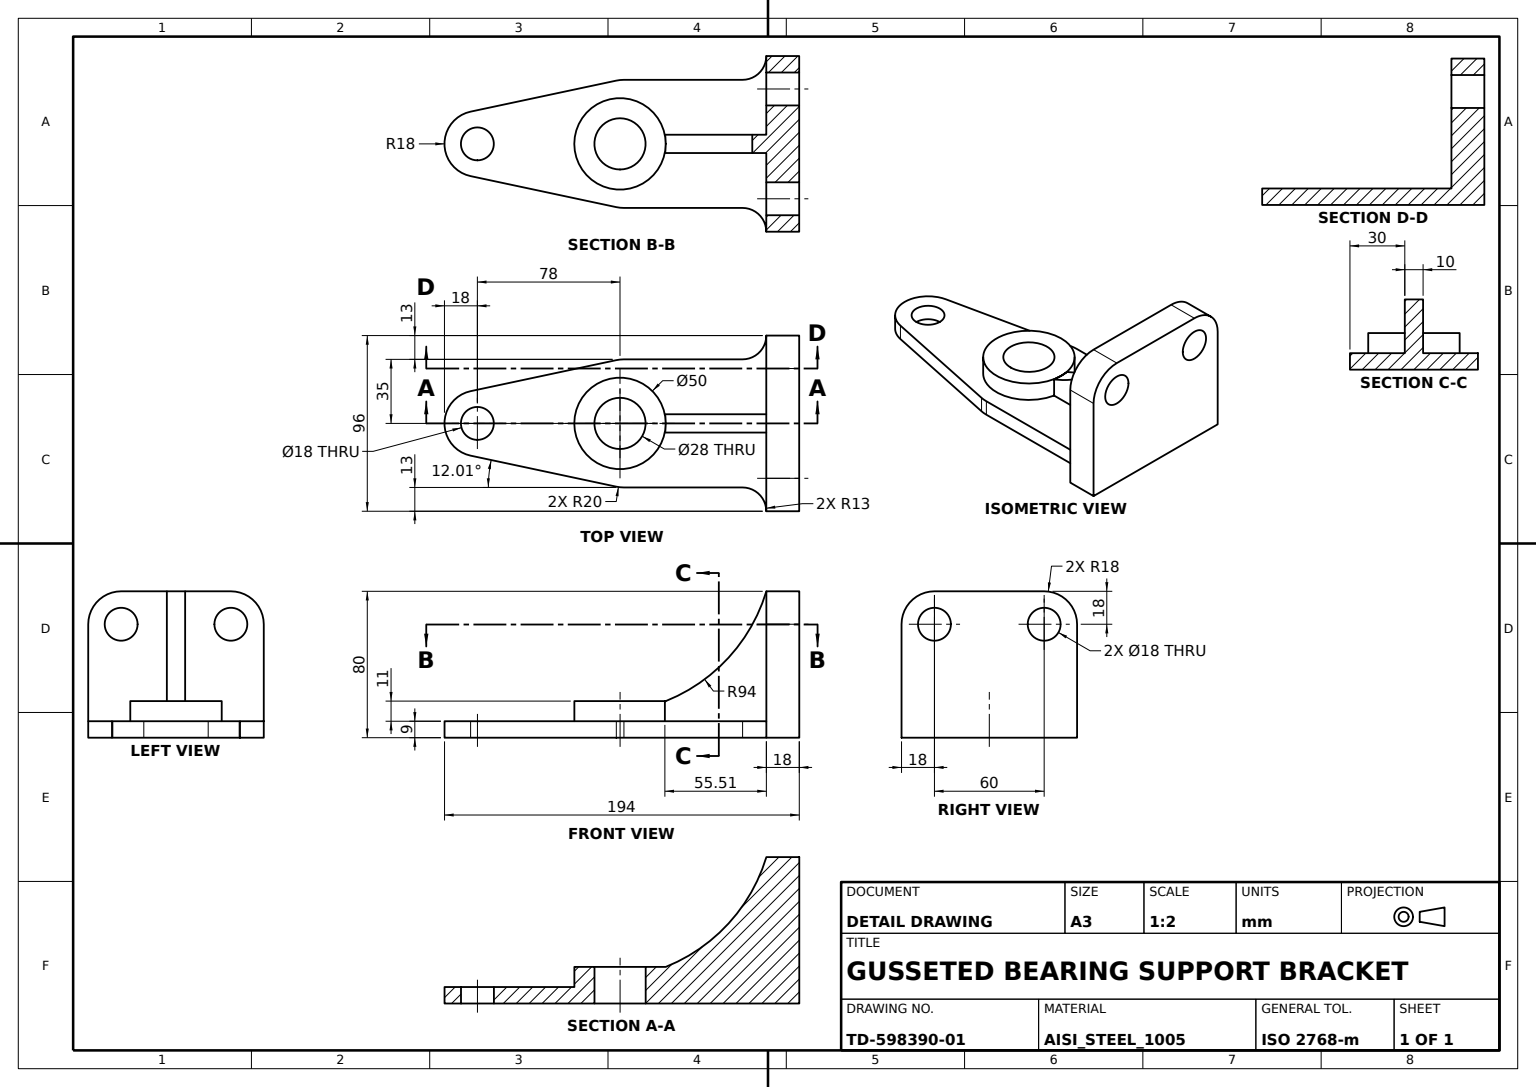
ISO-10303-21;
HEADER;
FILE_DESCRIPTION((''),'2;1');
FILE_NAME('','',(''),(''),'','','');
FILE_SCHEMA(('AUTOMOTIVE_DESIGN'));
ENDSEC;
DATA;
#1=APPLICATION_CONTEXT('');
#2=PRODUCT_CONTEXT('',#1,'mechanical');
#3=PRODUCT('','','',(#2));
#4=PRODUCT_DEFINITION_FORMATION('','',#3);
#5=PRODUCT_DEFINITION_CONTEXT('',#1,'design');
#6=PRODUCT_DEFINITION('','',#4,#5);
#7=PRODUCT_DEFINITION_SHAPE('','',#6);
#8=(LENGTH_UNIT()NAMED_UNIT(*)SI_UNIT(.MILLI.,.METRE.));
#9=(NAMED_UNIT(*)PLANE_ANGLE_UNIT()SI_UNIT($,.RADIAN.));
#10=(NAMED_UNIT(*)SI_UNIT($,.STERADIAN.)SOLID_ANGLE_UNIT());
#11=UNCERTAINTY_MEASURE_WITH_UNIT(LENGTH_MEASURE(0.005),#8,'distance_accuracy_value','');
#12=(GEOMETRIC_REPRESENTATION_CONTEXT(3)GLOBAL_UNCERTAINTY_ASSIGNED_CONTEXT((#11))GLOBAL_UNIT_ASSIGNED_CONTEXT((#8,#9,#10))REPRESENTATION_CONTEXT('',''));
#13=CARTESIAN_POINT('',(9.,0.,9.));
#14=VERTEX_POINT('',#13);
#15=CARTESIAN_POINT('',(0.,0.,9.));
#16=DIRECTION('',(0.,0.,1.));
#17=DIRECTION('',(1.,0.,0.));
#18=AXIS2_PLACEMENT_3D('',#15,#16,#17);
#19=CIRCLE('',#18,9.);
#20=EDGE_CURVE('',#14,#14,#19,.T.);
#21=ORIENTED_EDGE('',*,*,#20,.T.);
#22=EDGE_LOOP('',(#21));
#23=FACE_BOUND('',#22,.T.);
#24=CARTESIAN_POINT('',(9.,0.,0.));
#25=VERTEX_POINT('',#24);
#26=CARTESIAN_POINT('',(0.,0.,0.));
#27=AXIS2_PLACEMENT_3D('',#26,#16,#17);
#28=CIRCLE('',#27,9.);
#29=EDGE_CURVE('',#25,#25,#28,.T.);
#30=ORIENTED_EDGE('',*,*,#29,.F.);
#31=EDGE_LOOP('',(#30));
#32=FACE_BOUND('',#31,.T.);
#33=DIRECTION('',(0.,0.,-1.));
#34=DIRECTION('',(-1.,0.,0.));
#35=AXIS2_PLACEMENT_3D('',#15,#33,#34);
#36=CYLINDRICAL_SURFACE('',#35,9.);
#37=ADVANCED_FACE('',(#23,#32),#36,.F.);
#38=CARTESIAN_POINT('',(-5.,103.,20.));
#39=VERTEX_POINT('',#38);
#40=CARTESIAN_POINT('',(-5.,158.,80.));
#41=VERTEX_POINT('',#40);
#42=CARTESIAN_POINT('',(-5.,68.038419,107.256449));
#43=DIRECTION('',(0.,1.,0.));
#44=AXIS2_PLACEMENT_3D('',#42,#17,#43);
#45=CIRCLE('',#44,94.);
#46=EDGE_CURVE('',#39,#41,#45,.T.);
#47=ORIENTED_EDGE('',*,*,#46,.T.);
#48=CARTESIAN_POINT('',(-5.,158.,9.));
#49=VERTEX_POINT('',#48);
#50=CARTESIAN_POINT('',(-5.,158.,107.256449));
#51=VECTOR('',#16,1000.);
#52=LINE('',#50,#51);
#53=EDGE_CURVE('',#49,#41,#52,.T.);
#54=ORIENTED_EDGE('',*,*,#53,.F.);
#55=CARTESIAN_POINT('',(-5.,102.494897,9.));
#56=VERTEX_POINT('',#55);
#57=CARTESIAN_POINT('',(-5.,68.038419,9.));
#58=VECTOR('',#43,1000.);
#59=LINE('',#57,#58);
#60=EDGE_CURVE('',#56,#49,#59,.T.);
#61=ORIENTED_EDGE('',*,*,#60,.F.);
#62=CARTESIAN_POINT('',(-5.,102.494897,19.797617));
#63=VERTEX_POINT('',#62);
#64=CARTESIAN_POINT('',(-5.,102.494897,20.));
#65=VECTOR('',#33,1000.);
#66=LINE('',#64,#65);
#67=EDGE_CURVE('',#63,#56,#66,.T.);
#68=ORIENTED_EDGE('',*,*,#67,.F.);
#69=DIRECTION('',(0.,-0.928260095,-0.371931709));
#70=VECTOR('',#69,1000.);
#71=LINE('',#38,#70);
#72=EDGE_CURVE('',#39,#63,#71,.T.);
#73=ORIENTED_EDGE('',*,*,#72,.F.);
#74=EDGE_LOOP('',(#47,#54,#61,#68,#73));
#75=FACE_BOUND('',#74,.T.);
#76=AXIS2_PLACEMENT_3D('',#42,#17,#33);
#77=PLANE('',#76);
#78=ADVANCED_FACE('',(#75),#77,.F.);
#79=CARTESIAN_POINT('',(0.,103.,20.));
#80=VERTEX_POINT('',#79);
#81=CARTESIAN_POINT('',(5.,103.,20.));
#82=VECTOR('',#34,1000.);
#83=LINE('',#81,#82);
#84=EDGE_CURVE('',#80,#39,#83,.T.);
#85=ORIENTED_EDGE('',*,*,#84,.F.);
#86=VERTEX_POINT('',#81);
#87=EDGE_CURVE('',#86,#80,#83,.T.);
#88=ORIENTED_EDGE('',*,*,#87,.F.);
#89=CARTESIAN_POINT('',(5.,158.,80.));
#90=VERTEX_POINT('',#89);
#91=CARTESIAN_POINT('',(5.,68.038419,107.256449));
#92=AXIS2_PLACEMENT_3D('',#91,#17,#43);
#93=CIRCLE('',#92,94.);
#94=EDGE_CURVE('',#86,#90,#93,.T.);
#95=ORIENTED_EDGE('',*,*,#94,.T.);
#96=LINE('',#89,#82);
#97=EDGE_CURVE('',#90,#41,#96,.T.);
#98=ORIENTED_EDGE('',*,*,#97,.T.);
#99=ORIENTED_EDGE('',*,*,#46,.F.);
#100=EDGE_LOOP('',(#85,#88,#95,#98,#99));
#101=FACE_BOUND('',#100,.T.);
#102=AXIS2_PLACEMENT_3D('',#91,#34,#16);
#103=CYLINDRICAL_SURFACE('',#102,94.);
#104=ADVANCED_FACE('',(#101),#103,.F.);
#105=CARTESIAN_POINT('',(0.,78.,9.983095));
#106=DIRECTION('',(0.,0.371931709,-0.928260095));
#107=AXIS2_PLACEMENT_3D('',#105,#106,#69);
#108=ELLIPSE('',#107,26.932107,25.);
#109=EDGE_CURVE('',#80,#63,#108,.F.);
#110=ORIENTED_EDGE('',*,*,#109,.F.);
#111=ORIENTED_EDGE('',*,*,#84,.T.);
#112=ORIENTED_EDGE('',*,*,#72,.T.);
#113=EDGE_LOOP('',(#110,#111,#112));
#114=FACE_BOUND('',#113,.T.);
#115=DIRECTION('',(0.,0.928260095,0.371931709));
#116=AXIS2_PLACEMENT_3D('',#81,#106,#115);
#117=PLANE('',#116);
#118=ADVANCED_FACE('',(#114),#117,.F.);
#119=CARTESIAN_POINT('',(-17.605848,-3.746214,9.));
#120=VERTEX_POINT('',#119);
#121=CARTESIAN_POINT('',(-17.605848,-3.746214,0.));
#122=VERTEX_POINT('',#121);
#123=LINE('',#119,#65);
#124=EDGE_CURVE('',#120,#122,#123,.T.);
#125=ORIENTED_EDGE('',*,*,#124,.T.);
#126=CARTESIAN_POINT('',(17.605848,-3.746214,0.));
#127=VERTEX_POINT('',#126);
#128=AXIS2_PLACEMENT_3D('',#26,#33,#17);
#129=CIRCLE('',#128,18.);
#130=EDGE_CURVE('',#127,#122,#129,.T.);
#131=ORIENTED_EDGE('',*,*,#130,.F.);
#132=CARTESIAN_POINT('',(17.605848,-3.746214,9.));
#133=VERTEX_POINT('',#132);
#134=LINE('',#132,#65);
#135=EDGE_CURVE('',#133,#127,#134,.T.);
#136=ORIENTED_EDGE('',*,*,#135,.F.);
#137=AXIS2_PLACEMENT_3D('',#15,#33,#17);
#138=CIRCLE('',#137,18.);
#139=EDGE_CURVE('',#133,#120,#138,.T.);
#140=ORIENTED_EDGE('',*,*,#139,.T.);
#141=EDGE_LOOP('',(#125,#131,#136,#140));
#142=FACE_BOUND('',#141,.T.);
#143=CYLINDRICAL_SURFACE('',#35,18.);
#144=ADVANCED_FACE('',(#142),#143,.T.);
#145=CARTESIAN_POINT('',(48.,176.,0.));
#146=VERTEX_POINT('',#145);
#147=CARTESIAN_POINT('',(48.,158.,0.));
#148=VERTEX_POINT('',#147);
#149=DIRECTION('',(0.,-1.,0.));
#150=VECTOR('',#149,1000.);
#151=LINE('',#145,#150);
#152=EDGE_CURVE('',#146,#148,#151,.T.);
#153=ORIENTED_EDGE('',*,*,#152,.F.);
#154=CARTESIAN_POINT('',(48.,176.,62.));
#155=VERTEX_POINT('',#154);
#156=LINE('',#154,#65);
#157=EDGE_CURVE('',#155,#146,#156,.T.);
#158=ORIENTED_EDGE('',*,*,#157,.F.);
#159=CARTESIAN_POINT('',(48.,158.,62.));
#160=VERTEX_POINT('',#159);
#161=LINE('',#154,#150);
#162=EDGE_CURVE('',#155,#160,#161,.T.);
#163=ORIENTED_EDGE('',*,*,#162,.T.);
#164=CARTESIAN_POINT('',(48.,158.,9.));
#165=VERTEX_POINT('',#164);
#166=LINE('',#159,#65);
#167=EDGE_CURVE('',#160,#165,#166,.T.);
#168=ORIENTED_EDGE('',*,*,#167,.T.);
#169=LINE('',#164,#65);
#170=EDGE_CURVE('',#165,#148,#169,.T.);
#171=ORIENTED_EDGE('',*,*,#170,.T.);
#172=EDGE_LOOP('',(#153,#158,#163,#168,#171));
#173=FACE_BOUND('',#172,.T.);
#174=AXIS2_PLACEMENT_3D('',#154,#34,#16);
#175=PLANE('',#174);
#176=ADVANCED_FACE('',(#173),#175,.F.);
#177=ORIENTED_EDGE('',*,*,#67,.T.);
#178=CARTESIAN_POINT('',(5.,102.494897,9.));
#179=VERTEX_POINT('',#178);
#180=CARTESIAN_POINT('',(0.,78.,9.));
#181=AXIS2_PLACEMENT_3D('',#180,#33,#34);
#182=CIRCLE('',#181,25.);
#183=EDGE_CURVE('',#179,#56,#182,.T.);
#184=ORIENTED_EDGE('',*,*,#183,.F.);
#185=CARTESIAN_POINT('',(5.,102.494897,19.797617));
#186=VERTEX_POINT('',#185);
#187=CARTESIAN_POINT('',(5.,102.494897,20.));
#188=LINE('',#187,#65);
#189=EDGE_CURVE('',#179,#186,#188,.F.);
#190=ORIENTED_EDGE('',*,*,#189,.T.);
#191=EDGE_CURVE('',#186,#80,#108,.F.);
#192=ORIENTED_EDGE('',*,*,#191,.T.);
#193=CARTESIAN_POINT('',(0.,78.,20.));
#194=AXIS2_PLACEMENT_3D('',#193,#33,#17);
#195=CIRCLE('',#194,25.);
#196=EDGE_CURVE('',#80,#80,#195,.T.);
#197=ORIENTED_EDGE('',*,*,#196,.T.);
#198=ORIENTED_EDGE('',*,*,#109,.T.);
#199=EDGE_LOOP('',(#177,#184,#190,#192,#197,#198));
#200=FACE_BOUND('',#199,.T.);
#201=AXIS2_PLACEMENT_3D('',#193,#33,#34);
#202=CYLINDRICAL_SURFACE('',#201,25.);
#203=ADVANCED_FACE('',(#200),#202,.T.);
#204=CARTESIAN_POINT('',(30.,176.,80.));
#205=VERTEX_POINT('',#204);
#206=CARTESIAN_POINT('',(30.,158.,80.));
#207=VERTEX_POINT('',#206);
#208=LINE('',#204,#150);
#209=EDGE_CURVE('',#205,#207,#208,.T.);
#210=ORIENTED_EDGE('',*,*,#209,.T.);
#211=CARTESIAN_POINT('',(30.,158.,62.));
#212=AXIS2_PLACEMENT_3D('',#211,#43,#34);
#213=CIRCLE('',#212,18.);
#214=EDGE_CURVE('',#207,#160,#213,.T.);
#215=ORIENTED_EDGE('',*,*,#214,.T.);
#216=ORIENTED_EDGE('',*,*,#162,.F.);
#217=CARTESIAN_POINT('',(30.,176.,62.));
#218=AXIS2_PLACEMENT_3D('',#217,#43,#34);
#219=CIRCLE('',#218,18.);
#220=EDGE_CURVE('',#205,#155,#219,.T.);
#221=ORIENTED_EDGE('',*,*,#220,.F.);
#222=EDGE_LOOP('',(#210,#215,#216,#221));
#223=FACE_BOUND('',#222,.T.);
#224=AXIS2_PLACEMENT_3D('',#217,#149,#33);
#225=CYLINDRICAL_SURFACE('',#224,18.);
#226=ADVANCED_FACE('',(#223),#225,.T.);
#227=CARTESIAN_POINT('',(14.,78.,0.));
#228=VERTEX_POINT('',#227);
#229=CARTESIAN_POINT('',(0.,78.,0.));
#230=AXIS2_PLACEMENT_3D('',#229,#33,#17);
#231=CIRCLE('',#230,14.);
#232=EDGE_CURVE('',#228,#228,#231,.T.);
#233=ORIENTED_EDGE('',*,*,#232,.F.);
#234=EDGE_LOOP('',(#233));
#235=FACE_BOUND('',#234,.T.);
#236=CARTESIAN_POINT('',(-35.,80.104269,0.));
#237=VERTEX_POINT('',#236);
#238=CARTESIAN_POINT('',(-35.,145.,0.));
#239=VERTEX_POINT('',#238);
#240=LINE('',#236,#58);
#241=EDGE_CURVE('',#237,#239,#240,.T.);
#242=ORIENTED_EDGE('',*,*,#241,.T.);
#243=CARTESIAN_POINT('',(-48.,158.,0.));
#244=VERTEX_POINT('',#243);
#245=CARTESIAN_POINT('',(-48.,145.,0.));
#246=AXIS2_PLACEMENT_3D('',#245,#16,#17);
#247=CIRCLE('',#246,13.);
#248=EDGE_CURVE('',#239,#244,#247,.T.);
#249=ORIENTED_EDGE('',*,*,#248,.T.);
#250=CARTESIAN_POINT('',(-48.,176.,0.));
#251=VERTEX_POINT('',#250);
#252=LINE('',#250,#150);
#253=EDGE_CURVE('',#251,#244,#252,.T.);
#254=ORIENTED_EDGE('',*,*,#253,.F.);
#255=LINE('',#145,#82);
#256=EDGE_CURVE('',#146,#251,#255,.T.);
#257=ORIENTED_EDGE('',*,*,#256,.F.);
#258=ORIENTED_EDGE('',*,*,#152,.T.);
#259=CARTESIAN_POINT('',(35.,145.,0.));
#260=VERTEX_POINT('',#259);
#261=CARTESIAN_POINT('',(48.,145.,0.));
#262=AXIS2_PLACEMENT_3D('',#261,#16,#34);
#263=CIRCLE('',#262,13.);
#264=EDGE_CURVE('',#148,#260,#263,.T.);
#265=ORIENTED_EDGE('',*,*,#264,.T.);
#266=CARTESIAN_POINT('',(35.,80.104269,0.));
#267=VERTEX_POINT('',#266);
#268=LINE('',#259,#150);
#269=EDGE_CURVE('',#260,#267,#268,.T.);
#270=ORIENTED_EDGE('',*,*,#269,.T.);
#271=CARTESIAN_POINT('',(34.562053,75.941809,0.));
#272=VERTEX_POINT('',#271);
#273=CARTESIAN_POINT('',(15.,80.104269,0.));
#274=AXIS2_PLACEMENT_3D('',#273,#33,#34);
#275=CIRCLE('',#274,20.);
#276=EDGE_CURVE('',#267,#272,#275,.T.);
#277=ORIENTED_EDGE('',*,*,#276,.T.);
#278=DIRECTION('',(-0.20812299,-0.978102664,0.));
#279=VECTOR('',#278,1000.);
#280=LINE('',#271,#279);
#281=EDGE_CURVE('',#272,#127,#280,.T.);
#282=ORIENTED_EDGE('',*,*,#281,.T.);
#283=ORIENTED_EDGE('',*,*,#130,.T.);
#284=CARTESIAN_POINT('',(-34.562053,75.941809,0.));
#285=VERTEX_POINT('',#284);
#286=DIRECTION('',(-0.20812299,0.978102664,0.));
#287=VECTOR('',#286,1000.);
#288=LINE('',#121,#287);
#289=EDGE_CURVE('',#122,#285,#288,.T.);
#290=ORIENTED_EDGE('',*,*,#289,.T.);
#291=CARTESIAN_POINT('',(-15.,80.104269,0.));
#292=AXIS2_PLACEMENT_3D('',#291,#33,#17);
#293=CIRCLE('',#292,20.);
#294=EDGE_CURVE('',#285,#237,#293,.T.);
#295=ORIENTED_EDGE('',*,*,#294,.T.);
#296=EDGE_LOOP('',(#242,#249,#254,#257,#258,#265,#270,#277,#282,#283,#290,#295));
#297=FACE_BOUND('',#296,.T.);
#298=ORIENTED_EDGE('',*,*,#29,.T.);
#299=EDGE_LOOP('',(#298));
#300=FACE_BOUND('',#299,.T.);
#301=AXIS2_PLACEMENT_3D('',#26,#33,#34);
#302=PLANE('',#301);
#303=ADVANCED_FACE('',(#235,#297,#300),#302,.T.);
#304=ORIENTED_EDGE('',*,*,#232,.T.);
#305=EDGE_LOOP('',(#304));
#306=FACE_BOUND('',#305,.T.);
#307=CARTESIAN_POINT('',(14.,78.,20.));
#308=VERTEX_POINT('',#307);
#309=CIRCLE('',#194,14.);
#310=EDGE_CURVE('',#308,#308,#309,.T.);
#311=ORIENTED_EDGE('',*,*,#310,.F.);
#312=EDGE_LOOP('',(#311));
#313=FACE_BOUND('',#312,.T.);
#314=CYLINDRICAL_SURFACE('',#201,14.);
#315=ADVANCED_FACE('',(#306,#313),#314,.F.);
#316=CARTESIAN_POINT('',(21.,158.,62.));
#317=VERTEX_POINT('',#316);
#318=CIRCLE('',#212,9.);
#319=EDGE_CURVE('',#317,#317,#318,.T.);
#320=ORIENTED_EDGE('',*,*,#319,.T.);
#321=EDGE_LOOP('',(#320));
#322=FACE_BOUND('',#321,.T.);
#323=ORIENTED_EDGE('',*,*,#167,.F.);
#324=ORIENTED_EDGE('',*,*,#214,.F.);
#325=CARTESIAN_POINT('',(-30.,158.,80.));
#326=VECTOR('',#17,1000.);
#327=LINE('',#325,#326);
#328=EDGE_CURVE('',#90,#207,#327,.T.);
#329=ORIENTED_EDGE('',*,*,#328,.F.);
#330=CARTESIAN_POINT('',(5.,158.,9.));
#331=VERTEX_POINT('',#330);
#332=CARTESIAN_POINT('',(5.,158.,107.256449));
#333=LINE('',#332,#51);
#334=EDGE_CURVE('',#90,#331,#333,.F.);
#335=ORIENTED_EDGE('',*,*,#334,.T.);
#336=CARTESIAN_POINT('',(-48.,158.,9.));
#337=LINE('',#336,#326);
#338=EDGE_CURVE('',#331,#165,#337,.T.);
#339=ORIENTED_EDGE('',*,*,#338,.T.);
#340=EDGE_LOOP('',(#323,#324,#329,#335,#339));
#341=FACE_BOUND('',#340,.T.);
#342=CARTESIAN_POINT('',(-30.,158.,62.));
#343=AXIS2_PLACEMENT_3D('',#342,#43,#16);
#344=PLANE('',#343);
#345=ADVANCED_FACE('',(#322,#341),#344,.F.);
#346=ORIENTED_EDGE('',*,*,#124,.F.);
#347=CARTESIAN_POINT('',(-34.562053,75.941809,9.));
#348=VERTEX_POINT('',#347);
#349=LINE('',#119,#287);
#350=EDGE_CURVE('',#120,#348,#349,.T.);
#351=ORIENTED_EDGE('',*,*,#350,.T.);
#352=LINE('',#347,#65);
#353=EDGE_CURVE('',#348,#285,#352,.T.);
#354=ORIENTED_EDGE('',*,*,#353,.T.);
#355=ORIENTED_EDGE('',*,*,#289,.F.);
#356=EDGE_LOOP('',(#346,#351,#354,#355));
#357=FACE_BOUND('',#356,.T.);
#358=DIRECTION('',(-0.978102664,-0.20812299,0.));
#359=DIRECTION('',(0.20812299,-0.978102664,0.));
#360=AXIS2_PLACEMENT_3D('',#119,#358,#359);
#361=PLANE('',#360);
#362=ADVANCED_FACE('',(#357),#361,.T.);
#363=CARTESIAN_POINT('',(-35.,80.104269,9.));
#364=VERTEX_POINT('',#363);
#365=CARTESIAN_POINT('',(-35.,145.,9.));
#366=VERTEX_POINT('',#365);
#367=LINE('',#363,#58);
#368=EDGE_CURVE('',#364,#366,#367,.T.);
#369=ORIENTED_EDGE('',*,*,#368,.T.);
#370=LINE('',#365,#65);
#371=EDGE_CURVE('',#366,#239,#370,.T.);
#372=ORIENTED_EDGE('',*,*,#371,.T.);
#373=ORIENTED_EDGE('',*,*,#241,.F.);
#374=LINE('',#363,#65);
#375=EDGE_CURVE('',#364,#237,#374,.T.);
#376=ORIENTED_EDGE('',*,*,#375,.F.);
#377=EDGE_LOOP('',(#369,#372,#373,#376));
#378=FACE_BOUND('',#377,.T.);
#379=AXIS2_PLACEMENT_3D('',#363,#34,#149);
#380=PLANE('',#379);
#381=ADVANCED_FACE('',(#378),#380,.T.);
#382=CARTESIAN_POINT('',(35.,145.,9.));
#383=VERTEX_POINT('',#382);
#384=LINE('',#382,#65);
#385=EDGE_CURVE('',#383,#260,#384,.T.);
#386=ORIENTED_EDGE('',*,*,#385,.T.);
#387=ORIENTED_EDGE('',*,*,#264,.F.);
#388=ORIENTED_EDGE('',*,*,#170,.F.);
#389=CARTESIAN_POINT('',(48.,145.,9.));
#390=AXIS2_PLACEMENT_3D('',#389,#16,#34);
#391=CIRCLE('',#390,13.);
#392=EDGE_CURVE('',#165,#383,#391,.T.);
#393=ORIENTED_EDGE('',*,*,#392,.T.);
#394=EDGE_LOOP('',(#386,#387,#388,#393));
#395=FACE_BOUND('',#394,.T.);
#396=AXIS2_PLACEMENT_3D('',#389,#33,#34);
#397=CYLINDRICAL_SURFACE('',#396,13.);
#398=ADVANCED_FACE('',(#395),#397,.F.);
#399=CARTESIAN_POINT('',(-48.,176.,62.));
#400=VERTEX_POINT('',#399);
#401=CARTESIAN_POINT('',(-30.,176.,80.));
#402=VERTEX_POINT('',#401);
#403=CARTESIAN_POINT('',(-30.,176.,62.));
#404=AXIS2_PLACEMENT_3D('',#403,#43,#34);
#405=CIRCLE('',#404,18.);
#406=EDGE_CURVE('',#400,#402,#405,.T.);
#407=ORIENTED_EDGE('',*,*,#406,.F.);
#408=CARTESIAN_POINT('',(-48.,158.,62.));
#409=VERTEX_POINT('',#408);
#410=LINE('',#399,#150);
#411=EDGE_CURVE('',#400,#409,#410,.T.);
#412=ORIENTED_EDGE('',*,*,#411,.T.);
#413=VERTEX_POINT('',#325);
#414=AXIS2_PLACEMENT_3D('',#342,#43,#34);
#415=CIRCLE('',#414,18.);
#416=EDGE_CURVE('',#409,#413,#415,.T.);
#417=ORIENTED_EDGE('',*,*,#416,.T.);
#418=LINE('',#401,#150);
#419=EDGE_CURVE('',#402,#413,#418,.T.);
#420=ORIENTED_EDGE('',*,*,#419,.F.);
#421=EDGE_LOOP('',(#407,#412,#417,#420));
#422=FACE_BOUND('',#421,.T.);
#423=AXIS2_PLACEMENT_3D('',#403,#149,#33);
#424=CYLINDRICAL_SURFACE('',#423,18.);
#425=ADVANCED_FACE('',(#422),#424,.T.);
#426=VERTEX_POINT('',#336);
#427=CARTESIAN_POINT('',(-48.,145.,9.));
#428=AXIS2_PLACEMENT_3D('',#427,#16,#17);
#429=CIRCLE('',#428,13.);
#430=EDGE_CURVE('',#366,#426,#429,.T.);
#431=ORIENTED_EDGE('',*,*,#430,.T.);
#432=LINE('',#336,#65);
#433=EDGE_CURVE('',#426,#244,#432,.T.);
#434=ORIENTED_EDGE('',*,*,#433,.T.);
#435=ORIENTED_EDGE('',*,*,#248,.F.);
#436=ORIENTED_EDGE('',*,*,#371,.F.);
#437=EDGE_LOOP('',(#431,#434,#435,#436));
#438=FACE_BOUND('',#437,.T.);
#439=AXIS2_PLACEMENT_3D('',#427,#33,#34);
#440=CYLINDRICAL_SURFACE('',#439,13.);
#441=ADVANCED_FACE('',(#438),#440,.F.);
#442=ORIENTED_EDGE('',*,*,#385,.F.);
#443=CARTESIAN_POINT('',(35.,80.104269,9.));
#444=VERTEX_POINT('',#443);
#445=LINE('',#382,#150);
#446=EDGE_CURVE('',#383,#444,#445,.T.);
#447=ORIENTED_EDGE('',*,*,#446,.T.);
#448=LINE('',#443,#65);
#449=EDGE_CURVE('',#444,#267,#448,.T.);
#450=ORIENTED_EDGE('',*,*,#449,.T.);
#451=ORIENTED_EDGE('',*,*,#269,.F.);
#452=EDGE_LOOP('',(#442,#447,#450,#451));
#453=FACE_BOUND('',#452,.T.);
#454=AXIS2_PLACEMENT_3D('',#382,#17,#43);
#455=PLANE('',#454);
#456=ADVANCED_FACE('',(#453),#455,.T.);
#457=CARTESIAN_POINT('',(34.562053,75.941809,9.));
#458=VERTEX_POINT('',#457);
#459=LINE('',#457,#279);
#460=EDGE_CURVE('',#458,#133,#459,.T.);
#461=ORIENTED_EDGE('',*,*,#460,.T.);
#462=ORIENTED_EDGE('',*,*,#135,.T.);
#463=ORIENTED_EDGE('',*,*,#281,.F.);
#464=LINE('',#457,#65);
#465=EDGE_CURVE('',#458,#272,#464,.T.);
#466=ORIENTED_EDGE('',*,*,#465,.F.);
#467=EDGE_LOOP('',(#461,#462,#463,#466));
#468=FACE_BOUND('',#467,.T.);
#469=DIRECTION('',(0.978102664,-0.20812299,0.));
#470=DIRECTION('',(0.20812299,0.978102664,0.));
#471=AXIS2_PLACEMENT_3D('',#457,#469,#470);
#472=PLANE('',#471);
#473=ADVANCED_FACE('',(#468),#472,.T.);
#474=ORIENTED_EDGE('',*,*,#310,.T.);
#475=EDGE_LOOP('',(#474));
#476=FACE_BOUND('',#475,.T.);
#477=ORIENTED_EDGE('',*,*,#196,.F.);
#478=EDGE_LOOP('',(#477));
#479=FACE_BOUND('',#478,.T.);
#480=PLANE('',#201);
#481=ADVANCED_FACE('',(#476,#479),#480,.F.);
#482=CARTESIAN_POINT('',(21.,176.,62.));
#483=VERTEX_POINT('',#482);
#484=CIRCLE('',#218,9.);
#485=EDGE_CURVE('',#483,#483,#484,.T.);
#486=ORIENTED_EDGE('',*,*,#485,.F.);
#487=EDGE_LOOP('',(#486));
#488=FACE_BOUND('',#487,.T.);
#489=ORIENTED_EDGE('',*,*,#220,.T.);
#490=ORIENTED_EDGE('',*,*,#157,.T.);
#491=ORIENTED_EDGE('',*,*,#256,.T.);
#492=LINE('',#250,#51);
#493=EDGE_CURVE('',#251,#400,#492,.T.);
#494=ORIENTED_EDGE('',*,*,#493,.T.);
#495=ORIENTED_EDGE('',*,*,#406,.T.);
#496=LINE('',#401,#326);
#497=EDGE_CURVE('',#402,#205,#496,.T.);
#498=ORIENTED_EDGE('',*,*,#497,.T.);
#499=EDGE_LOOP('',(#489,#490,#491,#494,#495,#498));
#500=FACE_BOUND('',#499,.T.);
#501=CARTESIAN_POINT('',(-21.,176.,62.));
#502=VERTEX_POINT('',#501);
#503=AXIS2_PLACEMENT_3D('',#403,#149,#17);
#504=CIRCLE('',#503,9.);
#505=EDGE_CURVE('',#502,#502,#504,.T.);
#506=ORIENTED_EDGE('',*,*,#505,.T.);
#507=EDGE_LOOP('',(#506));
#508=FACE_BOUND('',#507,.T.);
#509=AXIS2_PLACEMENT_3D('',#403,#43,#16);
#510=PLANE('',#509);
#511=ADVANCED_FACE('',(#488,#500,#508),#510,.T.);
#512=LINE('',#81,#70);
#513=EDGE_CURVE('',#86,#186,#512,.T.);
#514=ORIENTED_EDGE('',*,*,#513,.F.);
#515=ORIENTED_EDGE('',*,*,#87,.T.);
#516=ORIENTED_EDGE('',*,*,#191,.F.);
#517=EDGE_LOOP('',(#514,#515,#516));
#518=FACE_BOUND('',#517,.T.);
#519=ADVANCED_FACE('',(#518),#117,.F.);
#520=ORIENTED_EDGE('',*,*,#319,.F.);
#521=EDGE_LOOP('',(#520));
#522=FACE_BOUND('',#521,.T.);
#523=ORIENTED_EDGE('',*,*,#485,.T.);
#524=EDGE_LOOP('',(#523));
#525=FACE_BOUND('',#524,.T.);
#526=CYLINDRICAL_SURFACE('',#224,9.);
#527=ADVANCED_FACE('',(#522,#525),#526,.F.);
#528=ORIENTED_EDGE('',*,*,#449,.F.);
#529=CARTESIAN_POINT('',(15.,80.104269,9.));
#530=AXIS2_PLACEMENT_3D('',#529,#33,#34);
#531=CIRCLE('',#530,20.);
#532=EDGE_CURVE('',#444,#458,#531,.T.);
#533=ORIENTED_EDGE('',*,*,#532,.T.);
#534=ORIENTED_EDGE('',*,*,#465,.T.);
#535=ORIENTED_EDGE('',*,*,#276,.F.);
#536=EDGE_LOOP('',(#528,#533,#534,#535));
#537=FACE_BOUND('',#536,.T.);
#538=CYLINDRICAL_SURFACE('',#530,20.);
#539=ADVANCED_FACE('',(#537),#538,.T.);
#540=LINE('',#243,#51);
#541=EDGE_CURVE('',#426,#409,#540,.T.);
#542=ORIENTED_EDGE('',*,*,#541,.T.);
#543=ORIENTED_EDGE('',*,*,#411,.F.);
#544=ORIENTED_EDGE('',*,*,#493,.F.);
#545=ORIENTED_EDGE('',*,*,#253,.T.);
#546=ORIENTED_EDGE('',*,*,#433,.F.);
#547=EDGE_LOOP('',(#542,#543,#544,#545,#546));
#548=FACE_BOUND('',#547,.T.);
#549=AXIS2_PLACEMENT_3D('',#250,#17,#33);
#550=PLANE('',#549);
#551=ADVANCED_FACE('',(#548),#550,.F.);
#552=ORIENTED_EDGE('',*,*,#419,.T.);
#553=EDGE_CURVE('',#413,#41,#327,.T.);
#554=ORIENTED_EDGE('',*,*,#553,.T.);
#555=ORIENTED_EDGE('',*,*,#97,.F.);
#556=ORIENTED_EDGE('',*,*,#328,.T.);
#557=ORIENTED_EDGE('',*,*,#209,.F.);
#558=ORIENTED_EDGE('',*,*,#497,.F.);
#559=EDGE_LOOP('',(#552,#554,#555,#556,#557,#558));
#560=FACE_BOUND('',#559,.T.);
#561=AXIS2_PLACEMENT_3D('',#401,#33,#34);
#562=PLANE('',#561);
#563=ADVANCED_FACE('',(#560),#562,.F.);
#564=ORIENTED_EDGE('',*,*,#20,.F.);
#565=EDGE_LOOP('',(#564));
#566=FACE_BOUND('',#565,.T.);
#567=ORIENTED_EDGE('',*,*,#139,.F.);
#568=ORIENTED_EDGE('',*,*,#460,.F.);
#569=ORIENTED_EDGE('',*,*,#532,.F.);
#570=ORIENTED_EDGE('',*,*,#446,.F.);
#571=ORIENTED_EDGE('',*,*,#392,.F.);
#572=ORIENTED_EDGE('',*,*,#338,.F.);
#573=CARTESIAN_POINT('',(5.,68.038419,9.));
#574=LINE('',#573,#58);
#575=EDGE_CURVE('',#331,#179,#574,.F.);
#576=ORIENTED_EDGE('',*,*,#575,.T.);
#577=ORIENTED_EDGE('',*,*,#183,.T.);
#578=ORIENTED_EDGE('',*,*,#60,.T.);
#579=EDGE_CURVE('',#426,#49,#337,.T.);
#580=ORIENTED_EDGE('',*,*,#579,.F.);
#581=ORIENTED_EDGE('',*,*,#430,.F.);
#582=ORIENTED_EDGE('',*,*,#368,.F.);
#583=CARTESIAN_POINT('',(-15.,80.104269,9.));
#584=AXIS2_PLACEMENT_3D('',#583,#33,#17);
#585=CIRCLE('',#584,20.);
#586=EDGE_CURVE('',#348,#364,#585,.T.);
#587=ORIENTED_EDGE('',*,*,#586,.F.);
#588=ORIENTED_EDGE('',*,*,#350,.F.);
#589=EDGE_LOOP('',(#567,#568,#569,#570,#571,#572,#576,#577,#578,#580,#581,#582,#587,#588));
#590=FACE_BOUND('',#589,.T.);
#591=PLANE('',#35);
#592=ADVANCED_FACE('',(#566,#590),#591,.F.);
#593=ORIENTED_EDGE('',*,*,#94,.F.);
#594=ORIENTED_EDGE('',*,*,#513,.T.);
#595=ORIENTED_EDGE('',*,*,#189,.F.);
#596=ORIENTED_EDGE('',*,*,#575,.F.);
#597=ORIENTED_EDGE('',*,*,#334,.F.);
#598=EDGE_LOOP('',(#593,#594,#595,#596,#597));
#599=FACE_BOUND('',#598,.T.);
#600=AXIS2_PLACEMENT_3D('',#91,#17,#33);
#601=PLANE('',#600);
#602=ADVANCED_FACE('',(#599),#601,.T.);
#603=ORIENTED_EDGE('',*,*,#505,.F.);
#604=EDGE_LOOP('',(#603));
#605=FACE_BOUND('',#604,.T.);
#606=CARTESIAN_POINT('',(-21.,158.,62.));
#607=VERTEX_POINT('',#606);
#608=AXIS2_PLACEMENT_3D('',#342,#149,#17);
#609=CIRCLE('',#608,9.);
#610=EDGE_CURVE('',#607,#607,#609,.T.);
#611=ORIENTED_EDGE('',*,*,#610,.T.);
#612=EDGE_LOOP('',(#611));
#613=FACE_BOUND('',#612,.T.);
#614=CYLINDRICAL_SURFACE('',#423,9.);
#615=ADVANCED_FACE('',(#605,#613),#614,.F.);
#616=ORIENTED_EDGE('',*,*,#610,.F.);
#617=EDGE_LOOP('',(#616));
#618=FACE_BOUND('',#617,.T.);
#619=ORIENTED_EDGE('',*,*,#53,.T.);
#620=ORIENTED_EDGE('',*,*,#553,.F.);
#621=ORIENTED_EDGE('',*,*,#416,.F.);
#622=ORIENTED_EDGE('',*,*,#541,.F.);
#623=ORIENTED_EDGE('',*,*,#579,.T.);
#624=EDGE_LOOP('',(#619,#620,#621,#622,#623));
#625=FACE_BOUND('',#624,.T.);
#626=ADVANCED_FACE('',(#618,#625),#344,.F.);
#627=ORIENTED_EDGE('',*,*,#353,.F.);
#628=ORIENTED_EDGE('',*,*,#586,.T.);
#629=ORIENTED_EDGE('',*,*,#375,.T.);
#630=ORIENTED_EDGE('',*,*,#294,.F.);
#631=EDGE_LOOP('',(#627,#628,#629,#630));
#632=FACE_BOUND('',#631,.T.);
#633=AXIS2_PLACEMENT_3D('',#583,#33,#34);
#634=CYLINDRICAL_SURFACE('',#633,20.);
#635=ADVANCED_FACE('',(#632),#634,.T.);
#636=CLOSED_SHELL('',(#37,#78,#104,#118,#144,#176,#203,#226,#303,#315,#345,#362,#381,#398,#425,#441,#456,#473,#481,#511,#519,#527,#539,#551,#563,#592,#602,#615,#626,#635));
#637=MANIFOLD_SOLID_BREP('',#636);
#638=ADVANCED_BREP_SHAPE_REPRESENTATION('',(#637),#12);
#639=SHAPE_DEFINITION_REPRESENTATION(#7,#638);
ENDSEC;
END-ISO-10303-21;
